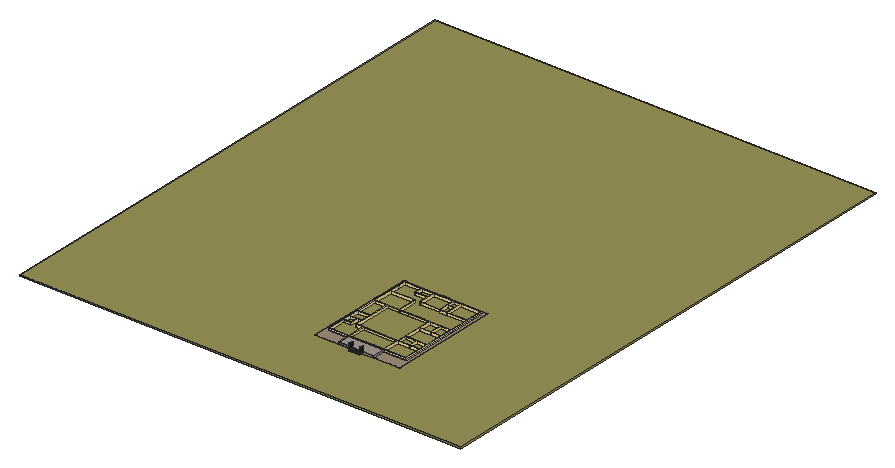
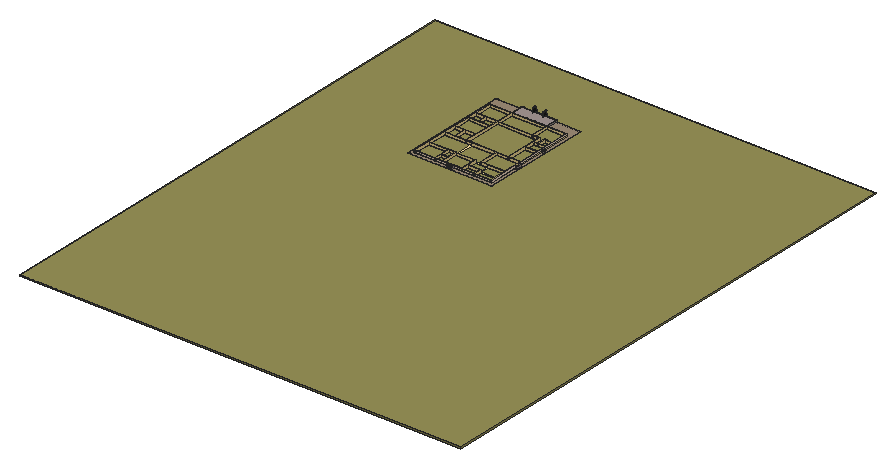
# SketchUp Ruby script. Lengths in inches.
U = 1.inch
M = Sketchup.active_model
def pt(a) = Geom::Point3d.new(a.map { |v| v * U })
def face(e, loops, mat)
  f = e.add_face(loops[0].map { |a| pt(a) })
  loops[1..].each { |l| e.add_face(l.map { |a| pt(a) }).erase! }
  f.material = f.back_material = mat if mat
  f
end
# faces: each face lists its corners as indices into pts; further lists are holes
def faces(e, pts, list, mat = nil) = list.each { |f| face(e, (f[0].is_a?(Array) ? f : [f]).map { |l| l.map { |i| pts[i] } }, mat) }
# xy, xz, yz: faces in a plane at the given z, y or x. An outline is a flat list of corners, or four numbers for a rectangle; further outlines are holes
def ring(l) = l.size == 4 ? [[l[0], l[1]], [l[2], l[1]], [l[2], l[3]], [l[0], l[3]]] : l.each_slice(2).to_a
def flat(e, list, mat, &to3) = list.each { |f| face(e, (f[0].is_a?(Array) ? f : [f]).map { |l| ring(l).map { |u, v| to3.(u, v) } }, mat) }
def xy(e, z, list, mat = nil) = flat(e, list, mat) { |x, y| [x, y, z] }
def xz(e, y, list, mat = nil) = flat(e, list, mat) { |x, z| [x, y, z] }
def yz(e, x, list, mat = nil) = flat(e, list, mat) { |y, z| [x, y, z] }
def lines(e, pts, list) = list.each { |a, b| e.add_line(pt(pts[a]), pt(pts[b])) }
# prism: a flat outline (further loops are holes) pulled along v
def prism(e, loops, v, mat = nil)
  f = face(e, loops, mat); d = Geom::Vector3d.new(v.map { |x| x * U })
  f.pushpull(f.normal.samedirection?(d) ? d.length : -d.length)
end
def box(e, o, s, mat = nil) = prism(e, [[o, [o[0] + s[0], o[1], o[2]], [o[0] + s[0], o[1] + s[1], o[2]], [o[0], o[1] + s[1], o[2]]]], [0, 0, s[2]], mat)
def at(x, y, z, deg = 0) = Geom::Transformation.translation(pt([x, y, z])) * Geom::Transformation.rotation(ORIGIN, Z_AXIS, deg.degrees)
def axes(o, x, y, z) = Geom::Transformation.new([*x, 0, *y, 0, *z, 0, *pt(o).to_a, 1])
def part(name) = M.definitions.add(name)
# library, detail: a bought-in or finely detailed component or shape, given as its bounding box
def library(name, o, s) = part(name).tap { |d| box(d.entities, o, s) }
def detail(e, o, s) = box(e.add_group.entities, o, s)
def put(e, d, t, mat = nil) = e.add_instance(d, t).tap { |i| i.material = mat if mat }
def group(e, t, mat = nil) = e.add_group.tap { |g| g.transformation = t; g.material = mat if mat }.entities
root = M.entities
M.materials.add("Brick_20_1K").color = [126, 109, 93]
M.materials.add("C01_Vanilla_Cream").color = [255, 230, 206]
M.materials.add("D02_Buttercup_Glow").color = [255, 229, 155]
M.materials.add("M08_Obsidian_Black").color = [30, 30, 30]
M.materials.add("Marble_01_1K").color = [230, 221, 211]
M.materials.add("Marble_06_1K").color = [165, 150, 147]
M.materials.add("Plaster_02_1K").color = [157, 140, 119]
M.materials.add("Soil_04_1K").color = [152, 146, 88]
xy(root,12,[[[2754.29,659.69,2754.29,686.69,2398.48,686.69,2398.48,1787.69,3244.48,1787.69,3244.48,686.69,2865.42,686.69,2865.42,659.69],[2434.48,806.69,3208.48,806.69,3208.48,1751.69,2857.48,1751.69,2857.48,1777.07,2809.48,1777.07,2809.48,1751.69,2434.48,1751.69,2434.48,1460.46,2404.48,1460.46,2404.48,1412.46,2434.48,1412.46,2434.48,1133.3,2416.48,1133.3,2416.48,1097.3,2434.48,1097.3]],[[2434.48,806.69,3208.48,1751.69],[2569.48,989.69,2983.48,1373.69],[2641.48,815.69,2977.48,983.69],[2935.48,1379.69,3199.48,1571.69],[2443.48,1379.69,2683.48,1571.69],[2689.48,1379.69,2929.48,1571.69],[2983.48,815.69,3199.48,983.69],[2443.48,815.69,2635.48,815.69,2635.48,983.69,2563.48,983.69,2563.48,1061.69,2521.48,1061.69,2521.48,983.69,2443.48,983.69],[2989.48,1079.69,3199.48,1247.69],[3007.48,1577.69,3199.48,1745.69],[2737.48,1577.69,2929.48,1745.69],[2443.48,1169.69,2563.48,1373.69],[2443.48,1577.69,2605.48,1667.69],[2989.48,1253.69,3097.48,1373.69],[2443.48,1673.69,2605.48,1745.69],[2443.48,1067.69,2563.48,1163.69],[3103.48,1253.69,3199.48,1373.69],[2611.48,1577.69,2731.48,1667.69],[2989.48,989.69,3097.48,1073.69],[2611.48,1673.69,2731.48,1745.69],[3103.48,989.69,3199.48,1073.69],[2935.48,1577.69,3001.48,1667.69],[2443.48,989.69,2515.48,1061.69],[2935.48,1673.69,3001.48,1745.69]],[2416.48,1097.3,2434.48,1133.3],[2404.48,1412.46,2434.48,1460.46],[2809.48,1751.69,2857.48,1777.07]],"D02_Buttercup_Glow")
xy(root,17,[[2754.29,659.69,2865.42,668.69]],"Marble_06_1K")
xy(root,18,[[2754.29,659.69,2865.42,668.69]],"Marble_01_1K")
xy(root,18,[[2398.48,686.69,2635.48,686.69,2635.48,806.69,2434.48,806.69,2434.48,1751.69,3208.48,1751.69,3208.48,806.69,2983.48,806.69,2983.48,686.69,3244.48,686.69,3244.48,1787.69,2398.48,1787.69]],"Plaster_02_1K")
xy(root,18.4375,[[2404.48,1412.46,2414.42,1460.46]],"Marble_06_1K")
xy(root,23,[[2754.29,668.69,2865.42,677.69]],"Marble_06_1K")
xy(root,24,[[2754.29,668.69,2865.42,677.69]],"Marble_01_1K")
xy(root,24,[[2416.48,1097.3,2425.48,1133.3],[2809.48,1769.38,2857.48,1777.07]],"Marble_06_1K")
xy(root,29,[[2754.29,677.69,2865.42,686.69]],"Marble_06_1K")
xy(root,30,[[2754.29,677.69,2865.42,686.69]],"Marble_01_1K")
xy(root,30,[[2425.48,1097.3,2434.48,1133.3],[2414.42,1412.46,2424.79,1460.46],[2809.48,1761.69,2857.48,1769.38]],"Marble_06_1K")
xy(root,35,[[2635.48,686.69,2983.48,806.69]],"Marble_06_1K")
xz(root,659.69,[[2754.29,17,2865.42,18]],"Marble_01_1K")
xz(root,659.69,[[2754.29,12,2865.42,17]],"Marble_06_1K")
xz(root,668.69,[[2754.29,23,2865.42,24]],"Marble_01_1K")
xz(root,668.69,[[2754.29,17,2865.42,18],[2754.29,18,2865.42,23]],"Marble_06_1K")
xz(root,677.69,[[2754.29,29,2865.42,30]],"Marble_01_1K")
xz(root,677.69,[[2754.29,23,2865.42,24],[2754.29,24,2865.42,29]],"Marble_06_1K")
xz(root,686.69,[[2635.48,35,2983.48,36]],"Marble_01_1K")
xz(root,686.69,[[2865.42,12,2983.48,12,2983.48,35,2635.48,35,2635.48,18,2754.29,18,2754.29,30,2865.42,30],[2754.29,29,2865.42,30]],"Marble_06_1K")
xz(root,686.69,[[2398.48,12,2754.29,18],[2983.48,12,3244.48,18]],"Plaster_02_1K")
xz(root,806.69,[[2434.48,18,2635.48,36],[2983.48,18,3208.48,36]],"C01_Vanilla_Cream")
xz(root,806.69,[[2434.48,12,3208.48,12,3208.48,18,2983.48,18,2983.48,35,2635.48,35,2635.48,18,2434.48,18],[2773.48,35,2845.48,36]],"D02_Buttercup_Glow")
xz(root,806.69,[[2635.48,35,2773.48,36],[2845.48,35,2983.48,36]],"Marble_06_1K")
xz(root,815.69,[[2443.48,12,2635.48,36],[2641.48,12,2977.48,36],[2983.48,12,3199.48,36]],"D02_Buttercup_Glow")
xz(root,983.69,[[2443.48,12,2521.48,36],[2563.48,12,2635.48,36],[2641.48,12,2977.48,36],[2983.48,12,3199.48,36]],"D02_Buttercup_Glow")
xz(root,989.69,[[2443.48,12,2515.48,36],[2569.48,12,2983.48,36],[2989.48,12,3097.48,36],[3103.48,12,3199.48,36]],"D02_Buttercup_Glow")
xz(root,1061.69,[[2443.48,12,2515.48,36],[2521.48,12,2563.48,36]],"D02_Buttercup_Glow")
xz(root,1067.69,[[2443.48,12,2563.48,36]],"D02_Buttercup_Glow")
xz(root,1073.69,[[2989.48,12,3097.48,36],[3103.48,12,3199.48,36]],"D02_Buttercup_Glow")
xz(root,1079.69,[[2989.48,12,3199.48,36]],"D02_Buttercup_Glow")
xz(root,1097.3,[[2416.48,12,2434.48,24],[2425.48,24,2434.48,30]],"Marble_06_1K")
xz(root,1133.3,[[2416.48,12,2434.48,24],[2425.48,24,2434.48,30]],"Marble_06_1K")
xz(root,1163.69,[[2443.48,12,2563.48,36]],"D02_Buttercup_Glow")
xz(root,1169.69,[[2443.48,12,2563.48,36]],"D02_Buttercup_Glow")
xz(root,1247.69,[[2989.48,12,3199.48,36]],"D02_Buttercup_Glow")
xz(root,1253.69,[[2989.48,12,3097.48,36],[3103.48,12,3199.48,36]],"D02_Buttercup_Glow")
xz(root,1373.69,[[2443.48,12,2563.48,36],[2569.48,12,2983.48,36],[2989.48,12,3097.48,36],[3103.48,12,3199.48,36]],"D02_Buttercup_Glow")
xz(root,1379.69,[[2443.48,12,2683.48,36],[2689.48,12,2929.48,36],[2935.48,12,3199.48,36]],"D02_Buttercup_Glow")
xz(root,1412.46,[[2404.48,12,2434.48,12,2434.48,36,2424.79,36,2424.79,30,2414.42,30,2414.42,18.4375,2404.48,18.4375]],"Marble_06_1K")
xz(root,1460.46,[[2404.48,12,2404.48,18.4375,2414.42,18.4375,2414.42,30,2424.79,30,2424.79,36,2434.48,36,2434.48,12]],"Marble_06_1K")
xz(root,1571.69,[[2443.48,12,2683.48,36],[2935.48,12,3199.48,36]],"D02_Buttercup_Glow")
xz(root,1577.69,[[2443.48,12,2605.48,36],[2737.48,12,2929.48,36],[2935.48,12,3001.48,36],[3007.48,12,3199.48,36]],"D02_Buttercup_Glow")
xz(root,1667.69,[[2611.48,12,2731.48,36],[2935.48,12,3001.48,36]],"D02_Buttercup_Glow")
xz(root,1673.69,[[2611.48,12,2731.48,36],[2935.48,12,3001.48,36]],"D02_Buttercup_Glow")
xz(root,1745.69,[[2443.48,12,2605.48,36],[2611.48,12,2731.48,36],[2737.48,12,2929.48,36],[2935.48,12,3001.48,36],[3007.48,12,3199.48,36]],"D02_Buttercup_Glow")
xz(root,1751.69,[[2434.48,18,2809.48,36],[2857.48,18,3208.48,36]],"C01_Vanilla_Cream")
xz(root,1751.69,[[2434.48,12,2809.48,18],[2809.48,12,2857.48,18],[2857.48,12,3208.48,18]],"D02_Buttercup_Glow")
xz(root,1761.69,[[2809.48,30,2857.48,36]],"Marble_06_1K")
xz(root,1769.38,[[2809.48,24,2857.48,30]],"Marble_06_1K")
xz(root,1777.07,[[2809.48,12,2857.48,24]],"Marble_06_1K")
xz(root,1787.69,[[2398.48,12,3244.48,18]],"Plaster_02_1K")
yz(root,2398.48,[[686.69,12,1787.69,18]],"Plaster_02_1K")
yz(root,2404.48,[[1412.46,12,1460.46,18.4375]],"Marble_06_1K")
yz(root,2414.42,[[1412.46,18.4375,1460.46,30]],"Marble_06_1K")
yz(root,2416.48,[[1097.3,12,1133.3,24]],"Marble_06_1K")
yz(root,2424.79,[[1412.46,30,1460.46,36]],"Marble_06_1K")
yz(root,2425.48,[[1097.3,24,1133.3,30]],"Marble_06_1K")
yz(root,2434.48,[[806.69,18,1097.3,36],[1133.3,18,1412.46,36],[1460.46,18,1751.69,36]],"C01_Vanilla_Cream")
yz(root,2434.48,[[806.69,12,1097.3,18],[1097.3,12,1133.3,18],[1133.3,12,1412.46,18],[1412.46,12,1460.46,18],[1460.46,12,1751.69,18]],"D02_Buttercup_Glow")
yz(root,2434.48,[[1097.3,30,1133.3,36]],"Marble_06_1K")
yz(root,2443.48,[[815.69,12,983.69,36],[989.69,12,1061.69,36],[1067.69,12,1163.69,36],[1169.69,12,1373.69,36],[1379.69,12,1571.69,36],
  [1577.69,12,1667.69,36],[1673.69,12,1745.69,36]],"D02_Buttercup_Glow")
yz(root,2515.48,[[989.69,12,1061.69,36]],"D02_Buttercup_Glow")
yz(root,2521.48,[[983.69,12,1061.69,36]],"D02_Buttercup_Glow")
yz(root,2563.48,[[983.69,12,1061.69,36],[1067.69,12,1163.69,36],[1169.69,12,1373.69,36]],"D02_Buttercup_Glow")
yz(root,2569.48,[[989.69,12,1373.69,36]],"D02_Buttercup_Glow")
yz(root,2605.48,[[1673.69,12,1745.69,36]],"D02_Buttercup_Glow")
yz(root,2611.48,[[1673.69,12,1745.69,36]],"D02_Buttercup_Glow")
yz(root,2635.48,[[815.69,12,983.69,36]],"D02_Buttercup_Glow")
yz(root,2635.48,[[686.69,18,806.69,35],[686.69,35,806.69,36]],"Marble_06_1K")
yz(root,2641.48,[[815.69,12,983.69,36]],"D02_Buttercup_Glow")
yz(root,2683.48,[[1379.69,12,1571.69,36]],"D02_Buttercup_Glow")
yz(root,2689.48,[[1379.69,12,1571.69,36]],"D02_Buttercup_Glow")
yz(root,2731.48,[[1577.69,12,1667.69,36],[1673.69,12,1745.69,36]],"D02_Buttercup_Glow")
yz(root,2737.48,[[1577.69,12,1745.69,36]],"D02_Buttercup_Glow")
yz(root,2754.29,[[659.69,12,659.69,17,668.69,17,668.69,23,677.69,23,677.69,29,686.69,29,686.69,12],[659.69,17,668.69,18],[668.69,23,677.69,24],[677.69,29,686.69,30]],"Marble_06_1K")
yz(root,2809.48,[[1751.69,12,1751.69,36,1761.69,36,1761.69,30,1769.38,30,1769.38,24,1777.07,24,1777.07,12]],"Marble_06_1K")
yz(root,2857.48,[[1751.69,12,1777.07,12,1777.07,24,1769.38,24,1769.38,30,1761.69,30,1761.69,36,1751.69,36]],"Marble_06_1K")
yz(root,2865.42,[[659.69,12,686.69,12,686.69,29,677.69,29,677.69,23,668.69,23,668.69,17,659.69,17],[659.69,17,668.69,18],[668.69,23,677.69,24],[677.69,29,686.69,30]],"Marble_06_1K")
yz(root,2929.48,[[1577.69,12,1745.69,36]],"D02_Buttercup_Glow")
yz(root,2935.48,[[1577.69,12,1667.69,36],[1673.69,12,1745.69,36]],"D02_Buttercup_Glow")
yz(root,2977.48,[[815.69,12,983.69,36]],"D02_Buttercup_Glow")
yz(root,2983.48,[[815.69,12,983.69,36],[989.69,12,1373.69,36]],"D02_Buttercup_Glow")
yz(root,2983.48,[[686.69,18,806.69,35],[686.69,35,806.69,36]],"Marble_06_1K")
yz(root,2989.48,[[989.69,12,1073.69,36],[1079.69,12,1247.69,36],[1253.69,12,1373.69,36]],"D02_Buttercup_Glow")
yz(root,3001.48,[[1577.69,12,1667.69,36],[1673.69,12,1745.69,36]],"D02_Buttercup_Glow")
yz(root,3007.48,[[1577.69,12,1745.69,36]],"D02_Buttercup_Glow")
yz(root,3097.48,[[989.69,12,1073.69,36],[1253.69,12,1373.69,36]],"D02_Buttercup_Glow")
yz(root,3103.48,[[989.69,12,1073.69,36],[1253.69,12,1373.69,36]],"D02_Buttercup_Glow")
yz(root,3199.48,[[815.69,12,983.69,36],[989.69,12,1073.69,36],[1079.69,12,1247.69,36],[1253.69,12,1373.69,36],[1379.69,12,1571.69,36],
  [1577.69,12,1745.69,36]],"D02_Buttercup_Glow")
yz(root,3208.48,[[806.69,18,1751.69,36]],"C01_Vanilla_Cream")
yz(root,3208.48,[[806.69,12,1746.1,18],[1746.1,12,1751.69,18]],"D02_Buttercup_Glow")
yz(root,3244.48,[[686.69,12,1787.69,18]],"Plaster_02_1K")
p = [[2929.48,1571.69,12],[2929.48,1571.69,36],[2605.48,1667.69,12],[2605.48,1667.69,36],[2611.48,1577.69,12],[2611.48,1577.69,36]]
lines(root,p,[[0,1],[2,3],[4,5]])
g1 = group(root,at(1349.5625,0,0))
box(g1,[-1349.5625,0,0],[4396.5,5183.3125,12],"Soil_04_1K")
g2 = group(root,at(2754.29,686.69,36),"Brick_20_1K")
xy(g2,-18,[[0,-27,7,-9.29]],"M08_Obsidian_Black")
xy(g2,-6,[[0,-9.29,7,13.81]],"M08_Obsidian_Black")
xy(g2,34,[[0,-18,7,13.81]],"M08_Obsidian_Black")
xy(g2,34,[[-1,-19,7,-18],[-1,-18,0,13.81]],"Marble_01_1K")
xy(g2,36.69,[[-1,-19,7,13.81]],"Marble_01_1K")
xz(g2,-27,[[0,-18,7,4.35]],"M08_Obsidian_Black")
xz(g2,-19,[[-1,34,7,36.69]],"Marble_01_1K")
xz(g2,-18,[[0,10.34,7,34]],"M08_Obsidian_Black")
xz(g2,-9.29,[[0,-18,7,-6]],"M08_Obsidian_Black")
xz(g2,13.81,[[0,-6,7,34]],"M08_Obsidian_Black")
xz(g2,13.81,[[-1,34,7,36.69]],"Marble_01_1K")
yz(g2,-1,[[-19,34,13.81,36.69]],"Marble_01_1K")
yz(g2,0,[[-27,-18,-27,4.35,-18,10.34,-18,34,13.81,34,13.81,-6,-9.29,-6,-9.29,-18]],"M08_Obsidian_Black")
yz(g2,7,[[-27,-18,-9.29,-18,-9.29,-6,13.81,-6,13.81,34,-18,34,-18,10.34,-27,4.35]],"M08_Obsidian_Black")
yz(g2,7,[[-19,34,13.81,36.69]],"Marble_01_1K")
p = [[7,-27,4.35],[7,-18,10.34],[0,-18,10.34],[0,-27,4.35]]
faces(g2,p,[[0,1,2,3]],"M08_Obsidian_Black")
g3 = group(root,at(2858.42,686.69,36),"Brick_20_1K")
xy(g3,-18,[[0,-27,7,-9.29]],"M08_Obsidian_Black")
xy(g3,-6,[[0,-9.29,7,14.5]],"M08_Obsidian_Black")
xy(g3,34,[[0,-18,7,14.5]],"M08_Obsidian_Black")
xy(g3,34,[[-1,-19,0,14.5],[0,-19,7,-18],[7,-19,8,14.5]],"Marble_01_1K")
xy(g3,36,[[-1,-19,8,14.5]],"Marble_01_1K")
xz(g3,-27,[[0,-18,7,4.35]],"M08_Obsidian_Black")
xz(g3,-19,[[-1,34,8,36]],"Marble_01_1K")
xz(g3,-18,[[0,10.34,7,34]],"M08_Obsidian_Black")
xz(g3,-9.29,[[0,-18,7,-6]],"M08_Obsidian_Black")
xz(g3,14.5,[[0,-6,7,34]],"M08_Obsidian_Black")
xz(g3,14.5,[[-1,34,8,36]],"Marble_01_1K")
yz(g3,-1,[[-19,34,14.5,36]],"Marble_01_1K")
yz(g3,0,[[-27,-18,-27,4.35,-18,10.34,-18,34,14.5,34,14.5,-6,-9.29,-6,-9.29,-18]],"M08_Obsidian_Black")
yz(g3,7,[[-27,-18,-9.29,-18,-9.29,-6,14.5,-6,14.5,34,-18,34,-18,10.34,-27,4.35]],"M08_Obsidian_Black")
yz(g3,8,[[-19,34,14.5,36]],"Marble_01_1K")
p = [[7,-27,4.35],[7,-18,10.34],[0,-18,10.34],[0,-27,4.35]]
faces(g3,p,[[0,1,2,3]],"M08_Obsidian_Black")
